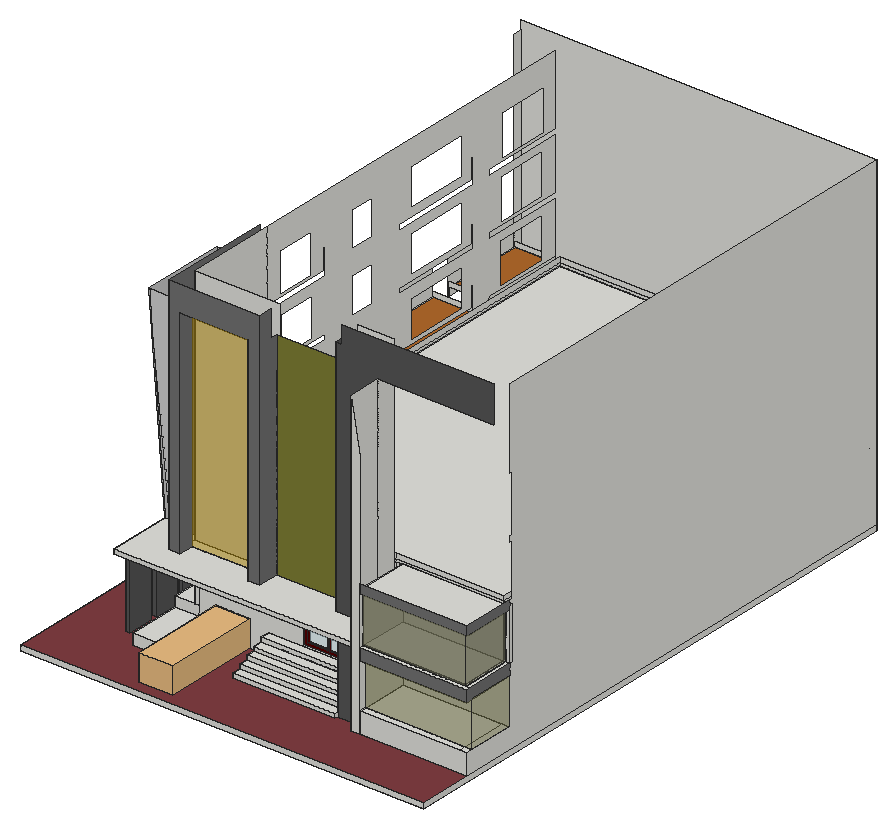
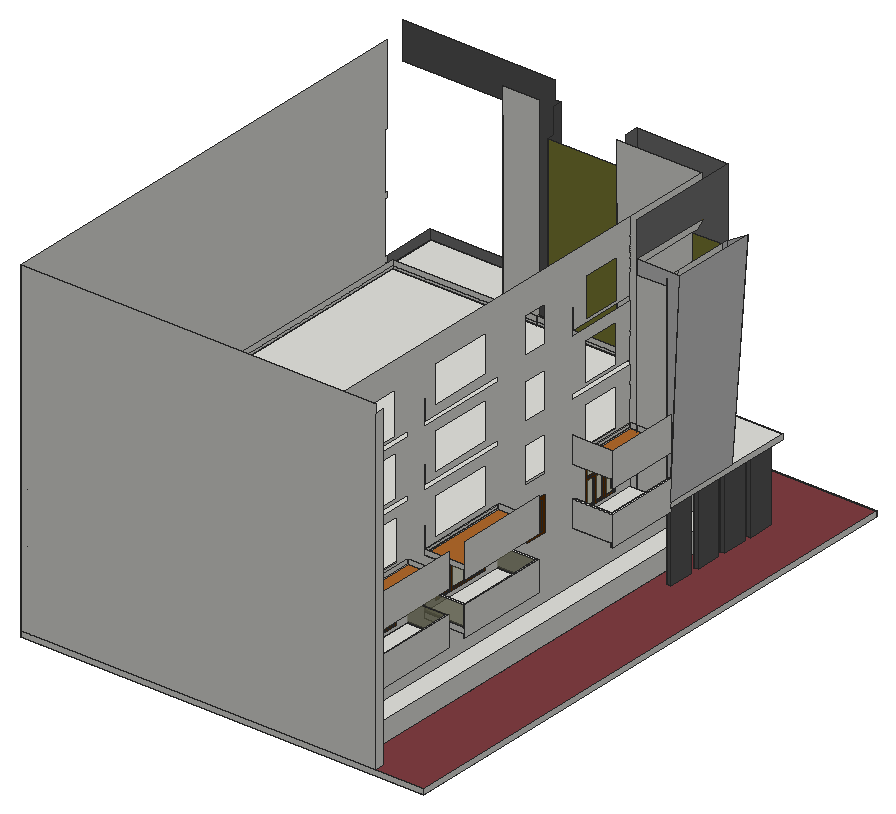
# SketchUp Ruby script. Lengths in inches.
U = 1.inch
M = Sketchup.active_model
def pt(a) = Geom::Point3d.new(a.map { |v| v * U })
def face(e, loops, mat)
  f = e.add_face(loops[0].map { |a| pt(a) })
  loops[1..].each { |l| e.add_face(l.map { |a| pt(a) }).erase! }
  f.material = f.back_material = mat if mat
  f
end
# faces: each face lists its corners as indices into pts; further lists are holes
def faces(e, pts, list, mat = nil) = list.each { |f| face(e, (f[0].is_a?(Array) ? f : [f]).map { |l| l.map { |i| pts[i] } }, mat) }
# xy, xz, yz: faces in a plane at the given z, y or x. An outline is a flat list of corners, or four numbers for a rectangle; further outlines are holes
def ring(l) = l.size == 4 ? [[l[0], l[1]], [l[2], l[1]], [l[2], l[3]], [l[0], l[3]]] : l.each_slice(2).to_a
def flat(e, list, mat, &to3) = list.each { |f| face(e, (f[0].is_a?(Array) ? f : [f]).map { |l| ring(l).map { |u, v| to3.(u, v) } }, mat) }
def xy(e, z, list, mat = nil) = flat(e, list, mat) { |x, y| [x, y, z] }
def xz(e, y, list, mat = nil) = flat(e, list, mat) { |x, z| [x, y, z] }
def yz(e, x, list, mat = nil) = flat(e, list, mat) { |y, z| [x, y, z] }
def lines(e, pts, list) = list.each { |a, b| e.add_line(pt(pts[a]), pt(pts[b])) }
# prism: a flat outline (further loops are holes) pulled along v
def prism(e, loops, v, mat = nil)
  f = face(e, loops, mat); d = Geom::Vector3d.new(v.map { |x| x * U })
  f.pushpull(f.normal.samedirection?(d) ? d.length : -d.length)
end
def box(e, o, s, mat = nil) = prism(e, [[o, [o[0] + s[0], o[1], o[2]], [o[0] + s[0], o[1] + s[1], o[2]], [o[0], o[1] + s[1], o[2]]]], [0, 0, s[2]], mat)
def at(x, y, z, deg = 0) = Geom::Transformation.translation(pt([x, y, z])) * Geom::Transformation.rotation(ORIGIN, Z_AXIS, deg.degrees)
def axes(o, x, y, z) = Geom::Transformation.new([*x, 0, *y, 0, *z, 0, *pt(o).to_a, 1])
def part(name) = M.definitions.add(name)
# library, detail: a bought-in or finely detailed component or shape, given as its bounding box
def library(name, o, s) = part(name).tap { |d| box(d.entities, o, s) }
def detail(e, o, s) = box(e.add_group.entities, o, s)
def put(e, d, t, mat = nil) = e.add_instance(d, t).tap { |i| i.material = mat if mat }
def group(e, t, mat = nil) = e.add_group.tap { |g| g.transformation = t; g.material = mat if mat }.entities
root = M.entities
M.materials.add("[Checkerboard Black]").color = [127, 127, 52]
M.materials.add("[Color A08]").color = [102, 50, 0]
M.materials.add("[Color A08]1").color = [84, 0, 0]
M.materials.add("[Color M02]").color = [198, 198, 198]
M.materials.add("[Color M05]").color = [114, 114, 114]
M.materials.add("[Color M06]").color = [86, 86, 86]
M.materials.add("[Concrete Stamped Ashlar]").color = [128, 61, 66]
M.materials.add("[Translucent Glass Blue]").color = [208, 160, 6]
M.materials["[Translucent Glass Blue]"].alpha = 0.5
M.materials.add("[Translucent Glass Gray]").color = [128, 128, 99]
M.materials["[Translucent Glass Gray]"].alpha = 0.5
M.materials.add("[Translucent Glass Gray]1").color = [128, 128, 95]
M.materials["[Translucent Glass Gray]1"].alpha = 0.5
M.materials.add("[Translucent Glass Gray]2").color = [128, 128, 74]
M.materials["[Translucent Glass Gray]2"].alpha = 0.5
M.materials.add("[Translucent Glass Safety]").color = [204, 235, 244]
M.materials["[Translucent Glass Safety]"].alpha = 0.5
M.materials.add("[Wood Bamboo]").color = [177, 105, 43]
c1 = library("custom el camino",[47.5625,9.86,-8],[222.64,79.59,60.9375])
c2 = part("Group\#1")
xy(c2.entities,0,[[0,0,10.1875,224.125]],"[Color A08]")
xy(c2.entities,8.5,[[0,8.5,10.1875,78.41],[0,83.11,10.1875,147.98],[0,152.67,10.1875,215.625]],"[Color A08]")
xy(c2.entities,168.57,[[0,8.5,10.1875,78.41],[0,83.11,10.1875,147.98],[0,152.67,10.1875,215.625]],"[Color A08]")
xy(c2.entities,174.05,[[0,8.5,10.1875,215.625]],"[Color A08]")
xy(c2.entities,240.6875,[[0,8.5,10.1875,215.625]],"[Color A08]")
xy(c2.entities,249.1875,[[0,0,10.1875,224.125]],"[Color A08]")
xz(c2.entities,0,[[0,0,10.1875,249.1875]],"[Color A08]")
xz(c2.entities,8.5,[[0,8.5,10.1875,168.57],[0,174.05,10.1875,240.6875]],"[Color A08]")
xz(c2.entities,78.41,[[0,8.5,10.1875,168.57]],"[Color A08]")
xz(c2.entities,83.11,[[0,8.5,10.1875,168.57]],"[Color A08]")
xz(c2.entities,147.98,[[0,8.5,10.1875,168.57]],"[Color A08]")
xz(c2.entities,152.67,[[0,8.5,10.1875,168.57]],"[Color A08]")
xz(c2.entities,215.625,[[0,8.5,10.1875,168.57],[0,174.05,10.1875,240.6875]],"[Color A08]")
xz(c2.entities,224.125,[[0,0,10.1875,249.1875]],"[Color A08]")
yz(c2.entities,0,[[[0,0,224.125,249.1875],[8.5,174.05,215.625,240.6875],[8.5,8.5,78.41,168.57],[83.11,8.5,147.98,168.57],[152.67,8.5,215.625,168.57]]],"[Color A08]")
yz(c2.entities,10.1875,[[[0,0,224.125,249.1875],[8.5,174.05,215.625,240.6875],[8.5,8.5,78.41,168.57],[83.11,8.5,147.98,168.57],[152.67,8.5,215.625,168.57]]],"[Color A08]")
yz(c2.entities,10.1875,[[8.5,8.5,78.41,168.57],[83.11,8.5,147.98,168.57],[152.67,8.5,215.625,168.57],[8.5,174.05,215.625,240.6875]],"[Translucent Glass Gray]1")
c3 = part("Group\#2")
xy(c3.entities,0,[[0,0,3.1875,51.25]],"[Color A08]")
xy(c3.entities,5.52,[[0,5.52,3.1875,45.73]],"[Color A08]")
xy(c3.entities,59.16,[[0,5.52,3.1875,45.73]],"[Color A08]")
xy(c3.entities,64.6875,[[0,0,3.1875,51.25]],"[Color A08]")
xz(c3.entities,0,[[0,0,3.1875,64.6875]],"[Color A08]")
xz(c3.entities,5.52,[[0,5.52,3.1875,59.16]],"[Color A08]")
xz(c3.entities,45.73,[[0,5.52,3.1875,59.16]],"[Color A08]")
xz(c3.entities,51.25,[[0,0,3.1875,64.6875]],"[Color A08]")
yz(c3.entities,0,[[[0,0,51.25,64.6875],[5.52,5.52,45.73,59.16]]],"[Color A08]")
yz(c3.entities,3.1875,[[[0,0,51.25,64.6875],[5.52,5.52,45.73,59.16]]],"[Color A08]")
yz(c3.entities,3.1875,[[5.52,5.52,45.73,59.16]],"[Translucent Glass Gray]1")
xy(root,0,[[0,0,206.0625,1311.875],[206.0625,0,933.8125,1311.875]])
xy(root,12,[[159.75,125.3125,215.0625,249.0625],[665.97,125.3125,686.75,134.3125],[686.75,125.3125,917.0625,134.3125],[917.0625,125.3125,933.8125,1292.9375],[665.97,134.3125,686.75,249.0625],
  [686.75,134.3125,917.0625,276.25],[376.3125,144.01,614.09,165.85],[614.09,150.875,665.97,249.0625],[376.3125,165.85,425.5625,249.0625],[425.5625,165.85,614.09,249.0625],
  [159.75,249.0625,159.75,1085.3125,215.0625,1085.3125,215.0625,1292.9375,917.0625,1292.9375,917.0625,276.25,686.75,276.25,686.75,249.0625],[111.0625,1289.125,206.0625,1311.875]])
xy(root,12,[[117.34,157.81,127.91,217.56],[117.34,235,127.91,292.37],[117.34,311.18,127.91,368.5],[117.34,390.68,127.91,447.37]],"[Color M06]")
xy(root,12,[[[0,0,933.8125,0,933.8125,125.3125,665.97,125.3125,665.97,150.875,614.09,150.875,614.09,144.01,376.3125,144.01,376.3125,249.0625,215.0625,249.0625,215.0625,125.3125,159.75,125.3125,159.75,1289.125,111.0625,1289.125,111.0625,1311.875,0,1311.875],[117.34,157.81,127.91,217.56],[117.34,235,127.91,292.37],[117.34,311.18,127.91,368.5],[117.34,390.68,127.91,447.37]]],"[Concrete Stamped Ashlar]")
xy(root,21.6,[[376.3125,144.01,614.09,165.85],[425.5625,165.85,614.09,187.69]])
xy(root,31.2,[[376.3125,165.85,614.09,185.62],[376.3125,185.62,614.09,187.69],[425.5625,187.69,614.09,207.46]])
xy(root,37.25,[[159.75,125.3125,215.0625,249.0625]])
xy(root,40.8,[[376.3125,185.62,614.09,205.38],[376.3125,205.38,614.09,207.46],[425.5625,207.46,614.09,227.22]])
xy(root,50.4,[[376.3125,205.38,614.09,227.22],[425.5625,227.22,614.09,249.0625]])
xy(root,60,[[686.75,125.3125,917.0625,141.125],[917.0625,125.3125,933.8125,141.125],[686.75,141.125,917.0625,249.0625],[917.0625,141.125,933.8125,249.0625],[376.3125,227.22,614.09,249.0625],
  [159.75,249.0625,206.0625,1289.125],[686.75,249.0625,917.0625,255.0625],[686.75,255.0625,917.0625,276.25]])
xy(root,63.17,[[458.56,249.0625,576.54,255.0625]])
xy(root,161.35,[[458.56,249.0625,576.54,255.0625]])
xy(root,165.25,[[922.0625,141.125,933.8125,249.0625]])
xy(root,165.25,[[686.75,124.9375,686.75,137.1875,922.0625,137.1875,922.0625,141.125,933.8125,141.125,933.8125,124.9375]],"[Color M05]")
xy(root,171.3125,[[111.0625,455.21,115.0625,624.125],[111.0625,838.07,115.0625,1052.01],[111.0625,1098.84,115.0625,1289.125]])
xy(root,180,[[623.97,133.1875,665.97,150.875],[686.75,137.1875,922.0625,141.125],[686.75,141.125,922.0625,249.0625],[614.09,150.875,665.97,249.0625]])
xy(root,180,[[[111.0625,133.1875,111.0625,455.21,115.0625,455.21,115.0625,624.125,206.0625,624.125,206.0625,249.0625,614.09,249.0625,614.09,150.875,623.97,150.875,623.97,133.1875],[117.34,235,127.91,292.37]],[115.0625,838.07,206.0625,1052.01],[115.0625,1098.84,206.0625,1289.125]],"[Wood Bamboo]")
xy(root,180.4375,[[117.34,390.68,127.91,447.37]],"[Color M06]")
xy(root,181.375,[[117.34,157.81,127.91,217.56]],"[Color M06]")
xy(root,183,[[215.0625,255.0625,917.0625,1292.9375]])
xy(root,185.9375,[[117.34,311.18,127.91,368.5]],"[Color M06]")
xy(root,192,[[686.75,124.9375,933.8125,133.1875],[111.0625,133.1875,665.97,133.1875,665.97,202.6875,568.625,202.6875,568.625,240.375,400.94,240.375,400.94,192.6875,374.07,192.6875,374.07,226.5,216.14,226.5,216.14,192.6875,189.6875,192.6875,189.6875,295.8125,121.48,295.8125,121.48,280.0625,111.0625,280.0625],[686.75,133.1875,686.75,137.1875,922.0625,137.1875,922.0625,249.0625,926.0625,249.0625,926.0625,133.1875],[926.0625,133.1875,933.8125,249.0625],[686.75,137.1875,922.0625,249.0625],
  [189.6875,192.6875,206.0625,455.21],[206.0625,192.6875,216.14,192.6875,216.14,226.5,374.07,226.5,374.07,192.6875,400.94,192.6875,400.94,249.0625,206.0625,249.0625],[568.625,202.6875,665.97,249.0625],[582.625,249.0625,665.97,255.0625],[215.0625,255.0625,917.0625,1292.9375],
  [111.0625,280.0625,121.48,422.4375],[121.48,295.8125,189.6875,455.21],[111.0625,422.4375,121.48,454.6875],[111.0625,454.6875,121.48,455.0625],[111.0625,455.0625,121.48,455.1875],
  [111.0625,455.1875,121.48,455.21],[116.95,455.21,206.0625,619.28],[115.0625,838.07,206.0625,842.07],[115.0625,842.07,206.0625,1048.01],[115.0625,1048.01,206.0625,1052.01],
  [115.0625,1098.84,206.0625,1102.84],[115.0625,1102.84,206.0625,1289.125]])
xy(root,196.65,[[206.0625,495.59,215.0625,585.34]])
xy(root,198.01,[[206.0625,1131.92,215.0625,1253.17]])
xy(root,199.4,[[206.0625,872.21,215.0625,1021.83]])
xy(root,201.97,[[206.0625,700.95,215.0625,757.76]])
xy(root,240,[[111.0625,455.1875,116.95,455.21],[111.0625,455.21,116.95,455.21,116.95,619.28,206.0625,619.28,206.0625,624.125,111.0625,624.125],[111.0625,838.07,115.0625,1052.01],[115.0625,838.07,206.0625,842.07],[115.0625,1048.01,206.0625,1052.01],
  [111.0625,1098.84,115.0625,1289.125],[115.0625,1098.84,206.0625,1102.84]])
xy(root,284.59,[[206.0625,700.95,215.0625,757.76]])
xy(root,285.84,[[206.0625,872.21,215.0625,1021.83]])
xy(root,286.4,[[206.0625,495.59,215.0625,585.34]])
xy(root,293.375,[[111.0625,455.21,115.0625,624.125],[111.0625,838.07,115.0625,1052.01],[111.0625,1098.84,115.0625,1289.125]])
xy(root,294.14,[[206.0625,1131.92,215.0625,1253.17]])
xy(root,302.75,[[686.75,124.9375,933.8125,133.1875],[926.0625,133.1875,933.8125,249.0625]],"[Color M05]")
xy(root,305.625,[[215.0625,255.0625,917.0625,1292.9375]])
xy(root,312,[[686.75,137.1875,922.0625,249.0625]])
xy(root,312,[[115.0625,455.21,206.0625,624.125],[115.0625,838.07,206.0625,1052.01],[115.0625,1098.84,206.0625,1289.125]],"[Wood Bamboo]")
xz(root,0,[[0,0,933.8125,12]])
xz(root,124.9375,[[686.75,165.25,933.8125,192],[686.75,302.75,933.8125,324]],"[Color M05]")
xz(root,125.3125,[[159.75,12,215.0625,37.25],[665.97,12,686.75,12,686.75,588,665.97,708],[686.75,12,933.8125,60]])
xz(root,133.1875,[[111.0625,180,665.97,192]])
xz(root,133.1875,[[686.75,192,926.0625,302.75]],"[Translucent Glass Gray]")
xz(root,137.1875,[[686.75,165.25,922.0625,180],[686.75,302.75,922.0625,312]])
xz(root,137.1875,[[686.75,192,922.0625,302.75]],"[Translucent Glass Gray]")
xz(root,141.125,[[686.75,60,933.8125,60,933.8125,165.25,922.0625,165.25,922.0625,180,686.75,180]],"[Translucent Glass Gray]2")
xz(root,144.01,[[376.3125,12,614.09,21.6]])
xz(root,150.875,[[614.09,12,665.97,180]],"[Color M06]")
xz(root,157.81,[[117.34,12,127.91,181.375]],"[Color M06]")
xz(root,165.85,[[425.5625,12,614.09,21.6],[376.3125,21.6,614.09,31.2]])
xz(root,185.62,[[376.3125,31.2,614.09,40.8]])
xz(root,187.69,[[425.5625,21.6,614.09,31.2]])
xz(root,192.6875,[[189.6875,192,216.14,192,216.14,691.09,374.07,691.09,374.07,192,400.94,192,400.94,750.75,189.6875,750.75]],"[Color M05]")
xz(root,202.6875,[[568.625,192,665.97,192,665.97,708,933.8125,708,933.8125,792.25,582.625,792.25,582.625,750.75,568.625,750.75]],"[Color M06]")
xz(root,205.38,[[376.3125,40.8,614.09,50.4]])
xz(root,207.46,[[425.5625,31.2,614.09,40.8]])
xz(root,217.56,[[117.34,12,127.91,181.375]],"[Color M06]")
xz(root,226.5,[[216.14,192,374.07,691.09]],"[Translucent Glass Blue]")
xz(root,227.22,[[425.5625,40.8,614.09,50.4],[376.3125,50.4,614.09,60]])
xz(root,235,[[117.34,12,127.91,180]],"[Color M06]")
xz(root,240.375,[[400.94,192,568.625,691.09]],"[Checkerboard Black]")
xz(root,249.0625,[[[215.0625,12,376.3125,12,376.3125,60,614.09,60,614.09,180,215.0625,180],[458.56,63.17,576.54,161.35]],[376.3125,12,425.5625,50.4],[425.5625,12,614.09,50.4],[614.09,12,665.97,60],[665.97,12,686.75,60],
  [159.75,37.25,215.0625,60],[376.3125,50.4,614.09,60],[206.0625,60,215.0625,180],[614.09,60,665.97,180],[665.97,60,686.75,180],
  [686.75,60,686.75,180,922.0625,180,922.0625,165.25,933.8125,165.25,933.8125,60],[206.0625,192,400.94,750.75],[568.625,192,582.625,312],[582.625,192,665.97,771],[686.75,192,922.0625,312],
  [922.0625,192,926.0625,302.75],[926.0625,192,933.8125,302.75],[922.0625,302.75,933.8125,312],[568.625,312,582.625,324]])
xz(root,255.0625,[[[215.0625,60,917.0625,180],[458.56,63.17,576.54,161.35]],[215.0625,180,917.0625,183],[215.0625,183,917.0625,192],[215.0625,192,582.625,305.625],[582.625,192,665.97,305.625],
  [665.97,192,917.0625,305.625],[917.0625,192,933.8125,305.625],[215.0625,305.625,582.625,312],[582.625,305.625,665.97,312],[665.97,305.625,917.0625,312],
  [917.0625,305.625,933.8125,312],[215.0625,312,582.625,324],[582.625,312,665.97,324],[665.97,312,917.0625,324]])
xz(root,276.25,[[686.75,12,917.0625,60]])
xz(root,292.37,[[117.34,12,127.91,180]],"[Color M06]")
xz(root,295.8125,[[121.48,192,189.6875,653.32]],"[Checkerboard Black]")
xz(root,311.18,[[117.34,12,127.91,185.9375]],"[Color M06]")
xz(root,368.5,[[117.34,12,127.91,185.9375]],"[Color M06]")
xz(root,390.68,[[117.34,12,127.91,180.4375]],"[Color M06]")
xz(root,447.37,[[117.34,12,127.91,180.4375]],"[Color M06]")
xz(root,455.1875,[[111.0625,192.01,111.0625,240,90.2,669.38]])
xz(root,455.1875,[[111.0625,192,111.0625,240,90.2,669.38,189.6875,669.38,189.6875,636,121.48,636,121.48,192]],"[Color M02]")
xz(root,455.21,[[111.0625,171.3125,115.0625,180],[111.0625,192,116.95,240],[121.48,192,189.6875,312],[189.6875,192,206.0625,312],[111.0625,293.375,115.0625,293.375,115.0625,312,121.48,312,121.48,324,111.0625,324],
  [121.48,312,189.6875,324],[189.6875,312,206.0625,324]])
xz(root,495.59,[[206.0625,196.65,215.0625,286.4]])
xz(root,585.34,[[206.0625,196.65,215.0625,286.4]])
xz(root,619.28,[[116.95,192,206.0625,240]])
xz(root,624.125,[[111.0625,171.3125,111.0625,240,206.0625,240,206.0625,180,115.0625,180,115.0625,171.3125],[111.0625,293.375,111.0625,372,206.0625,372,206.0625,312,115.0625,312,115.0625,293.375]])
xz(root,700.95,[[206.0625,201.97,215.0625,284.59]])
xz(root,757.76,[[206.0625,201.97,215.0625,284.59]])
xz(root,838.07,[[111.0625,171.3125,115.0625,171.3125,115.0625,180,206.0625,180,206.0625,192,111.0625,192],[111.0625,192,115.0625,240],[111.0625,293.375,115.0625,293.375,115.0625,312,206.0625,312,206.0625,324,111.0625,324]])
xz(root,838.07,[[115.0625,192,206.0625,240]],"[Translucent Glass Gray]")
xz(root,842.07,[[115.0625,192,206.0625,240]],"[Translucent Glass Gray]")
xz(root,872.21,[[206.0625,199.4,215.0625,285.84]])
xz(root,1021.83,[[206.0625,199.4,215.0625,285.84]])
xz(root,1048.01,[[115.0625,192,206.0625,240]],"[Translucent Glass Gray]")
xz(root,1052.01,[[111.0625,171.3125,111.0625,192,206.0625,192,206.0625,180,115.0625,180,115.0625,171.3125],[111.0625,192,115.0625,240],[111.0625,293.375,111.0625,324,206.0625,324,206.0625,312,115.0625,312,115.0625,293.375]])
xz(root,1052.01,[[115.0625,192,206.0625,240]],"[Translucent Glass Gray]")
xz(root,1098.84,[[111.0625,171.3125,115.0625,171.3125,115.0625,180,206.0625,180,206.0625,192,111.0625,192],[111.0625,192,115.0625,240],[111.0625,293.375,115.0625,293.375,115.0625,312,206.0625,312,206.0625,324,111.0625,324]])
xz(root,1098.84,[[115.0625,192,206.0625,240]],"[Translucent Glass Gray]")
xz(root,1102.84,[[115.0625,192,206.0625,240]],"[Translucent Glass Gray]")
xz(root,1131.92,[[206.0625,198.01,215.0625,294.14]])
xz(root,1253.17,[[206.0625,198.01,215.0625,294.14]])
xz(root,1289.125,[[159.75,12,206.0625,60],[111.0625,171.3125,111.0625,192,206.0625,192,206.0625,180,115.0625,180,115.0625,171.3125],[111.0625,192,115.0625,240],[111.0625,293.375,111.0625,324,206.0625,324,206.0625,312,115.0625,312,115.0625,293.375]])
xz(root,1289.125,[[111.0625,12,159.75,12,159.75,60,206.0625,60,206.0625,180,115.0625,180,115.0625,171.3125,111.0625,171.3125],[115.0625,192,206.0625,192,206.0625,312,115.0625,312,115.0625,293.375,111.0625,293.375,111.0625,240,115.0625,240]],"[Wood Bamboo]")
xz(root,1292.9375,[[215.0625,12,917.0625,183],[215.0625,183,917.0625,192],[215.0625,192,917.0625,305.625],[215.0625,305.625,917.0625,312],[215.0625,312,917.0625,324]])
xz(root,1311.875,[[0,0,933.8125,12],[111.0625,12,933.8125,771]])
yz(root,0,[[0,0,1311.875,12]])
yz(root,111.0625,[[1289.125,12,1311.875,750.75],[455.21,171.3125,624.125,240],[838.07,171.3125,1052.01,240],[1098.84,171.3125,1289.125,240],[133.1875,180,455.21,192],
  [455.1875,192,455.21,198.4375],[455.1875,198.4375,455.21,200.14],[455.1875,200.14,455.21,234.61],[455.1875,234.61,455.21,235.34],[455.1875,235.34,455.21,237.13],
  [455.1875,237.13,455.21,239.2],[455.1875,239.2,455.21,240],[455.21,293.375,624.125,372],[838.07,293.375,1052.01,372],[1098.84,293.375,1289.125,372]])
yz(root,115.0625,[[455.21,171.3125,624.125,180],[838.07,171.3125,1052.01,180],[1098.84,171.3125,1289.125,180],[838.07,192,842.07,240],[842.07,192,1048.01,240],
  [1048.01,192,1052.01,240],[1098.84,192,1102.84,240],[1102.84,192,1289.125,240],[455.21,293.375,624.125,312],[838.07,293.375,1052.01,312],
  [1098.84,293.375,1289.125,312]])
yz(root,116.95,[[455.21,192,619.28,240],[455.1875,208.12,455.21,240]])
yz(root,117.34,[[157.81,12,217.56,181.375],[235,12,292.37,180],[311.18,12,368.5,185.9375],[390.68,12,447.37,180.4375]],"[Color M06]")
yz(root,121.48,[[295.8125,192,422.4375,653.32],[422.4375,192,454.6875,653.32],[455.1875,192,455.21,636]])
yz(root,121.48,[[280.0625,192,295.8125,653.32]],"[Color M02]")
yz(root,127.91,[[157.81,12,217.56,181.375],[235,12,292.37,180],[311.18,12,368.5,185.9375],[390.68,12,447.37,180.4375]],"[Color M06]")
yz(root,159.75,[[125.3125,12,125.3125,37.25,249.0625,37.25,249.0625,60,1289.125,60,1289.125,12]])
yz(root,189.6875,[[295.8125,192,295.8125,653.32,455.1875,653.32,455.1875,636,455.21,636,455.21,192]])
yz(root,189.6875,[[192.6875,192,192.6875,750.75,455.21,750.75,455.21,653.32,455.1875,653.32,455.1875,669.38,260.8,669.38,280.0625,653.32,295.8125,653.32,295.8125,192]],"[Color M05]")
yz(root,206.0625,[[[249.0625,60,249.0625,180,624.125,180,624.125,240,619.28,240,619.28,192,455.21,192,455.21,312,624.125,312,624.125,372,619.9,372,619.9,324,459.83,324,459.83,372,455.21,372,455.21,444,624.125,444,624.125,504,620.39,504,620.39,456,458.47,456,458.47,504,455.21,504,455.21,576,624.125,576,624.125,636,619.85,636,619.85,588,459.9,588,459.9,636,455.21,636,455.21,750.75,1289.125,750.75,1289.125,588,1102.84,588,1102.84,636,1098.84,636,1098.84,576,1289.125,576,1289.125,456,1102.84,456,1102.84,497.6875,1098.84,497.6875,1098.84,444,1289.125,444,1289.125,324,1102.84,324,1102.84,372,1098.84,372,1098.84,312,1289.125,312,1289.125,192,1102.84,192,1102.84,240,1098.84,240,1098.84,180,1289.125,180,1289.125,60],[872.21,199.4,1021.83,285.84],[872.21,332.84,1021.83,419.28],[872.21,468.03,1021.83,554.47],[872.21,607.03,1021.83,693.47],[1131.92,198.01,1253.17,294.14],[1132.12,329.92,1253.37,426.05],[1132.73,462.44,1253.98,558.57],[1136.9,593.81,1258.15,689.93],[495.59,196.65,585.34,286.4],[495.54,461.48,585.29,551.23],[495.59,328.22,585.34,417.97],[494.02,594.11,583.77,683.86],[700.95,201.97,757.76,284.59],[703.45,596.28,760.27,678.91],[703.45,458.84,760.27,541.47],[703.45,325.72,760.27,408.34],[838.07,180,1052.01,180,1052.01,240,1048.01,240,1048.01,192,842.07,192,842.07,240,838.07,240],[838.07,576,1052.01,576,1052.01,636,1048.01,636,1048.01,588,842.07,588,842.07,636,838.07,636],[838.07,312,1052.01,312,1052.01,372,1048.01,372,1048.01,324,842.07,324,842.07,372,838.07,372],[838.07,444,1052.01,444,1052.01,497.6875,1048.01,497.6875,1048.01,456,842.07,456,842.07,497.6875,838.07,497.6875]],[1098.84,180,1289.125,192],[249.0625,192,455.21,750.75],[619.28,192,624.125,240],[838.07,192,842.07,240],
  [1048.01,192,1052.01,240],[1098.84,192,1102.84,240],[1098.84,312,1289.125,324]])
yz(root,215.0625,[[125.3125,12,134.3125,37.25],[134.3125,12,249.0625,37.25],[255.0625,12,1292.9375,180],[255.0625,180,1292.9375,183],[255.0625,183,1292.9375,192],
  [[255.0625,192,1292.9375,305.625],[872.21,199.4,1021.83,285.84],[1131.92,198.01,1253.17,294.14],[495.59,196.65,585.34,286.4],[700.95,201.97,757.76,284.59]],[255.0625,305.625,1292.9375,312],[255.0625,312,1292.9375,324]])
yz(root,216.14,[[192.6875,192,226.5,691.09]],"[Color M05]")
yz(root,374.07,[[192.6875,192,226.5,691.09]],"[Color M05]")
yz(root,376.3125,[[144.01,12,144.01,21.6,165.85,21.6,165.85,31.2,185.62,31.2,185.62,40.8,205.38,40.8,205.38,50.4,227.22,50.4,227.22,60,249.0625,60,249.0625,12]])
yz(root,400.94,[[240.375,192,249.0625,617.75]])
yz(root,400.94,[[192.6875,192,240.375,192,240.375,691.09,223.8125,691.09,223.8125,750.75,192.6875,750.75]],"[Color M05]")
yz(root,425.5625,[[165.85,12,249.0625,12,249.0625,50.4,227.22,50.4,227.22,40.8,207.46,40.8,207.46,31.2,187.69,31.2,187.69,21.6,165.85,21.6]])
yz(root,458.56,[[249.0625,63.17,255.0625,161.35]])
yz(root,568.625,[[240.375,192,249.0625,312],[240.375,312,249.0625,324]])
yz(root,568.625,[[202.6875,192,202.6875,750.75,223.8125,750.75,223.8125,691.09,240.375,691.09,240.375,192]],"[Color M06]")
yz(root,576.54,[[249.0625,63.17,255.0625,161.35]])
yz(root,582.625,[[249.0625,192,255.0625,312],[249.0625,312,255.0625,324]])
yz(root,614.09,[[144.01,12,150.875,21.6],[150.875,12,165.85,21.6],[165.85,21.6,187.69,31.2],[185.62,31.2,207.46,40.8],[205.38,40.8,227.22,50.4],
  [227.22,50.4,249.0625,60]])
yz(root,614.09,[[[165.85,12,165.85,21.6,150.875,21.6,150.875,180,249.0625,180,249.0625,60,227.22,60,227.22,50.4,249.0625,50.4,249.0625,12],[185.62,31.2,207.46,40.8]]],"[Color M06]")
yz(root,665.97,[[125.3125,12,125.3125,708,202.6875,708,202.6875,192,133.1875,192,133.1875,180,150.875,180,150.875,12],[150.875,12,249.0625,180],[202.6875,192,249.0625,708]])
yz(root,686.75,[[125.3125,12,249.0625,60],[249.0625,12,276.25,60],[125.3125,60,141.125,60,141.125,180,137.1875,180,137.1875,165.25,125.3125,165.25],[141.125,60,249.0625,180],[124.9375,165.25,125.3125,180],
  [125.3125,165.25,137.1875,180],[124.9375,180,125.3125,192],[125.3125,192,133.1875,302.75],[133.1875,192,137.1875,302.75],[137.1875,192,249.0625,312],
  [124.9375,302.75,125.3125,324]])
yz(root,917.0625,[[255.0625,12,276.25,60],[276.25,12,1292.9375,60],[255.0625,60,1292.9375,180],[255.0625,180,1292.9375,183],[255.0625,183,1292.9375,192],
  [255.0625,192,1292.9375,305.625],[255.0625,305.625,1292.9375,312],[255.0625,312,1292.9375,324]])
yz(root,922.0625,[[137.1875,165.25,141.125,180],[141.125,165.25,249.0625,180],[137.1875,302.75,249.0625,312]])
yz(root,922.0625,[[137.1875,192,249.0625,302.75]],"[Translucent Glass Gray]")
yz(root,926.0625,[[133.1875,192,249.0625,302.75]],"[Translucent Glass Gray]")
yz(root,933.8125,[[0,0,1311.875,12],[125.3125,12,1311.875,12,1311.875,771,249.0625,771,249.0625,588,255.0625,588,255.0625,456,249.0625,456,249.0625,444,255.0625,444,255.0625,324,249.0625,324,249.0625,312,255.0625,312,255.0625,192,249.0625,192,249.0625,60,125.3125,60],[249.0625,192,255.0625,312]])
yz(root,933.8125,[[124.9375,165.25,249.0625,192],[124.9375,302.75,249.0625,324]],"[Color M05]")
yz(root,933.8125,[[141.125,60,249.0625,165.25]],"[Translucent Glass Gray]2")
p = [[90.2,260.8,669.38],[90.2,455.1875,669.38],[111.0625,455.1875,192.01],[111.0625,455.1875,192],[111.0625,455.0625,192],[111.0625,454.6875,192],
  [111.0625,422.4375,192],[111.0625,280.0625,192],[121.48,280.0625,192],[121.48,280.0625,653.32],[206.0625,1085.3125,180],[215.0625,1085.3125,180],
  [917.0625,1292.9375,180],[933.8125,1292.9375,180],[115.0625,455.21,312],[115.0625,455.1875,312],[917.0625,1311.875,192],[917.0625,1292.9375,192],
  [917.0625,1292.9375,312],[917.0625,1311.875,312],[376.3125,187.69,21.6],[425.5625,187.69,21.6],[376.3125,207.46,31.2],[425.5625,207.46,31.2],
  [376.3125,227.22,40.8],[425.5625,227.22,40.8]]
faces(root,p,[[0,1,2,3,4,5,6,7],[7,8,0],[9,0,8]],"[Color M02]")
lines(root,p,[[10,11],[12,13],[14,15],[16,17],[18,19],[20,21],[22,23],[24,25]])
put(root,c1,at(342.09,-21.14,20,90))
g1 = group(root,at(458.56,249.0625,63.17))
xy(g1,0,[[0,0,117.98,4.68]],"[Color A08]1")
xy(g1,6.82,[[8.2,0,54.71,4.68],[58.64,0,109.79,4.68]],"[Color A08]1")
xy(g1,91.37,[[8.2,0,54.71,4.68],[58.64,0,109.79,4.68]],"[Color A08]1")
xy(g1,98.1875,[[0,0,117.98,4.68]],"[Color A08]1")
xz(g1,0,[[[0,0,117.98,98.1875],[58.64,6.82,109.79,91.37],[8.2,6.82,54.71,91.37]]],"[Color A08]1")
xz(g1,4.68,[[[0,0,117.98,98.1875],[58.64,6.82,109.79,91.37],[8.2,6.82,54.71,91.37]]],"[Color A08]1")
xz(g1,4.68,[[8.2,6.82,54.71,91.37],[58.64,6.82,109.79,91.37]],"[Translucent Glass Safety]")
yz(g1,0,[[0,0,4.68,98.1875]],"[Color A08]1")
yz(g1,8.2,[[0,6.82,4.68,91.37]],"[Color A08]1")
yz(g1,54.71,[[0,6.82,4.68,91.37]],"[Color A08]1")
yz(g1,58.64,[[0,6.82,4.68,91.37]],"[Color A08]1")
yz(g1,109.79,[[0,6.82,4.68,91.37]],"[Color A08]1")
yz(g1,117.98,[[0,0,4.68,98.1875]],"[Color A08]1")
put(root,c2,axes([206.0625,495.59,196.65],[0.56448,0,0],[0,0.40045,0],[0,0,0.36017]))
put(root,c2,axes([206.0625,1131.92,198.01],[0.3,0,0],[0,0.54099,0],[0,0,0.38575]))
put(root,c2,axes([206.0625,872.21,199.4],[0.504,0,0],[0,0.6676,0],[0,0,0.34688]))
put(root,c3,axes([206.0625,700.95,200.9],[2.19,0,0],[0,1.10854,0],[0,0,1.27]))
